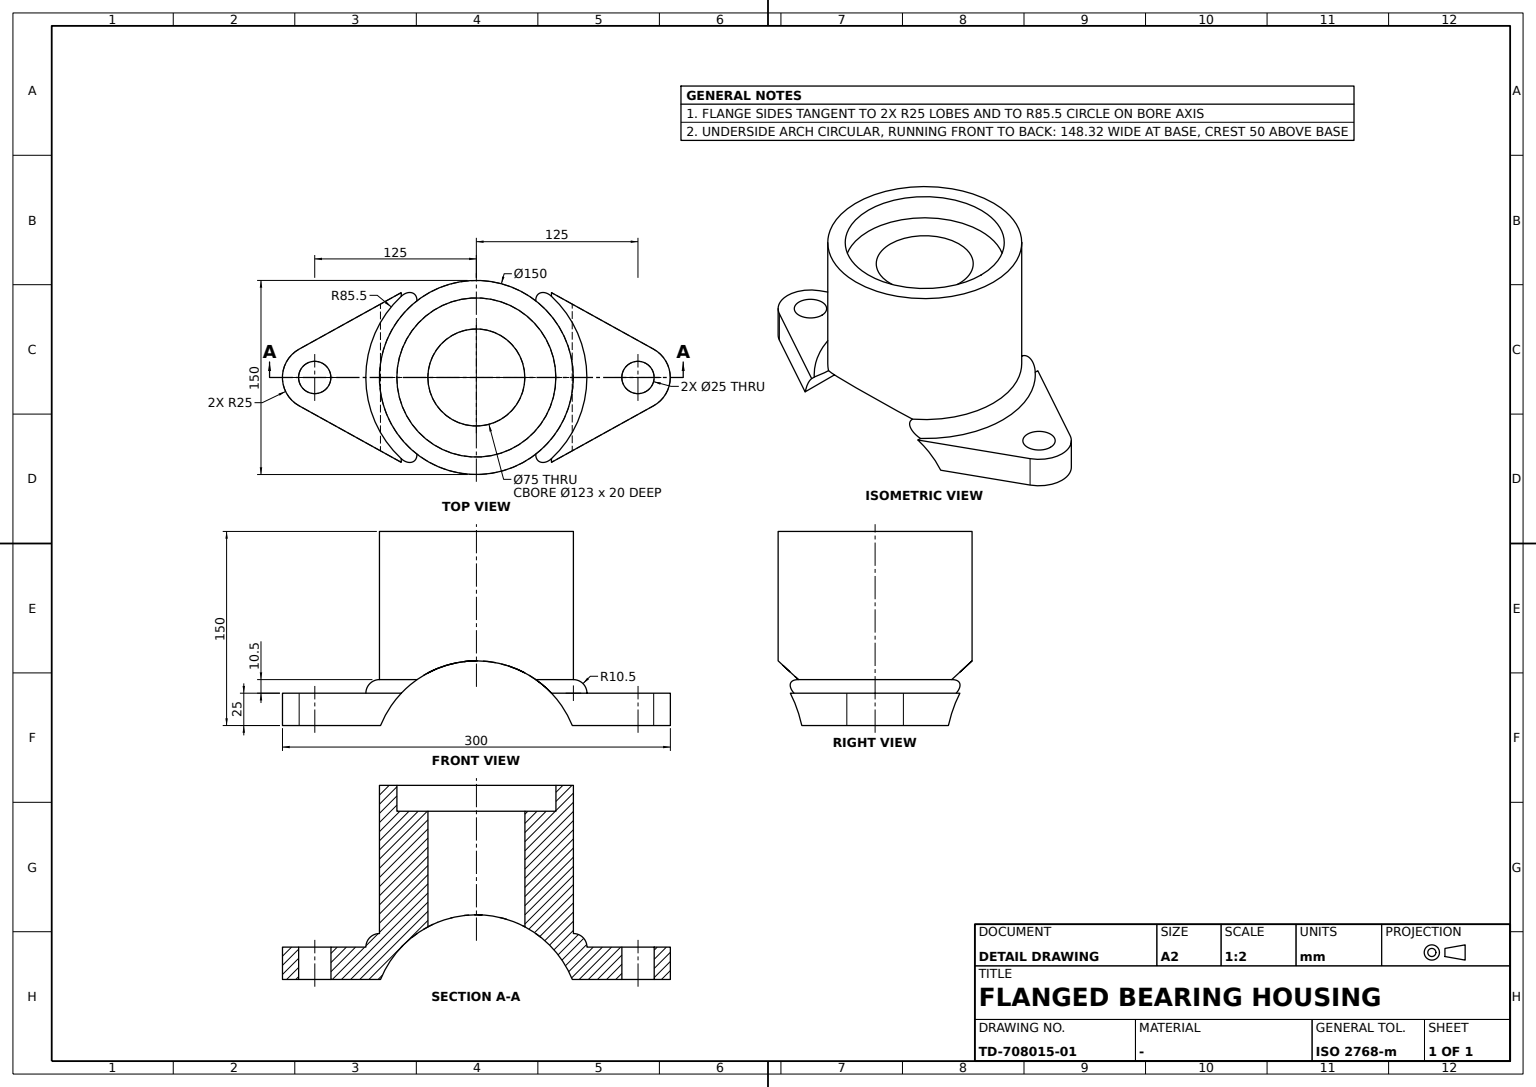
ISO-10303-21;
HEADER;
FILE_DESCRIPTION((''),'2;1');
FILE_NAME('','',(''),(''),'','','');
FILE_SCHEMA(('AUTOMOTIVE_DESIGN'));
ENDSEC;
DATA;
#1=APPLICATION_CONTEXT('');
#2=PRODUCT_CONTEXT('',#1,'mechanical');
#3=PRODUCT('','','',(#2));
#4=PRODUCT_DEFINITION_FORMATION('','',#3);
#5=PRODUCT_DEFINITION_CONTEXT('',#1,'design');
#6=PRODUCT_DEFINITION('','',#4,#5);
#7=PRODUCT_DEFINITION_SHAPE('','',#6);
#8=(LENGTH_UNIT()NAMED_UNIT(*)SI_UNIT(.MILLI.,.METRE.));
#9=(NAMED_UNIT(*)PLANE_ANGLE_UNIT()SI_UNIT($,.RADIAN.));
#10=(NAMED_UNIT(*)SI_UNIT($,.STERADIAN.)SOLID_ANGLE_UNIT());
#11=UNCERTAINTY_MEASURE_WITH_UNIT(LENGTH_MEASURE(1.E-05),#8,'distance_accuracy_value','');
#12=(GEOMETRIC_REPRESENTATION_CONTEXT(3)GLOBAL_UNCERTAINTY_ASSIGNED_CONTEXT((#11))GLOBAL_UNIT_ASSIGNED_CONTEXT((#8,#9,#10))REPRESENTATION_CONTEXT('',''));
#13=CARTESIAN_POINT('',(75.,0.,65.500023));
#14=VERTEX_POINT('',#13);
#15=CARTESIAN_POINT('',(45.932015,59.289544,65.500023));
#16=VERTEX_POINT('',#15);
#17=CARTESIAN_POINT('',(0.,0.,65.500023));
#18=DIRECTION('',(0.,0.,1.));
#19=DIRECTION('',(1.,0.,0.));
#20=AXIS2_PLACEMENT_3D('',#17,#18,#19);
#21=CIRCLE('',#20,75.);
#22=EDGE_CURVE('',#14,#16,#21,.T.);
#23=ORIENTED_EDGE('',*,*,#22,.T.);
#24=CARTESIAN_POINT('',(0.,74.999996,80.));
#25=VERTEX_POINT('',#24);
#26=CARTESIAN_POINT('',(44.42466,60.457302,66.557036));
#27=CARTESIAN_POINT('',(42.867243,61.587191,67.584494));
#28=CARTESIAN_POINT('',(41.259501,62.676771,68.579184));
#29=CARTESIAN_POINT('',(37.943975,64.769112,70.495736));
#30=CARTESIAN_POINT('',(34.432206,66.674154,72.251286));
#31=CARTESIAN_POINT('',(32.628216,67.576435,73.084976));
#32=CARTESIAN_POINT('',(28.788877,69.336495,74.71488));
#33=CARTESIAN_POINT('',(24.759204,70.848302,76.12074));
#34=CARTESIAN_POINT('',(22.623713,71.560134,76.783912));
#35=CARTESIAN_POINT('',(18.26572,72.83147,77.970027));
#36=CARTESIAN_POINT('',(13.757738,73.781552,78.858624));
#37=CARTESIAN_POINT('',(11.472246,74.17213,79.224278));
#38=CARTESIAN_POINT('',(7.811173,74.651918,79.673714));
#39=CARTESIAN_POINT('',(4.111316,74.906018,79.911892));
#40=CARTESIAN_POINT('',(2.741968,74.968674,79.970633));
#41=CARTESIAN_POINT('',(1.370943,74.999997,80.));
#42=B_SPLINE_CURVE_WITH_KNOTS('',5,(#15,#26,#27,#28,#29,#30,#31,#32,#33,#34,#35,#36,#37,#38,#39,#40,#41,#24),.UNSPECIFIED.,.F.,.F.,(6,3,3,3,3,6),(0.000015545,15.416004002,30.832008004,47.400792482,63.96957696,73.665798497),.UNSPECIFIED.);
#43=EDGE_CURVE('',#16,#25,#42,.T.);
#44=ORIENTED_EDGE('',*,*,#43,.T.);
#45=CARTESIAN_POINT('',(-35.956915,65.818692,71.463979));
#46=VERTEX_POINT('',#45);
#47=CARTESIAN_POINT('',(-3.005582,74.999994,80.));
#48=CARTESIAN_POINT('',(-6.010768,74.849434,79.858851));
#49=CARTESIAN_POINT('',(-8.997009,74.548401,79.576624));
#50=CARTESIAN_POINT('',(-13.856972,73.811882,78.886712));
#51=CARTESIAN_POINT('',(-18.575435,72.700605,77.84818));
#52=CARTESIAN_POINT('',(-20.404325,72.207987,77.388242));
#53=CARTESIAN_POINT('',(-24.004028,71.116214,76.370136));
#54=CARTESIAN_POINT('',(-27.477294,69.822077,75.166705));
#55=CARTESIAN_POINT('',(-29.179745,69.127095,74.521442));
#56=CARTESIAN_POINT('',(-31.57301,68.064182,73.536419));
#57=CARTESIAN_POINT('',(-33.889508,66.913561,72.473425));
#58=CARTESIAN_POINT('',(-34.586075,66.556124,72.143525));
#59=CARTESIAN_POINT('',(-35.275165,66.191134,71.807));
#60=B_SPLINE_CURVE_WITH_KNOTS('',5,(#24,#47,#48,#49,#50,#51,#52,#53,#54,#55,#56,#57,#58,#59,#45),.UNSPECIFIED.,.F.,.F.,(6,3,3,3,6),(73.665798497,94.92327613,108.689934936,122.456593742,128.461425552),.UNSPECIFIED.);
#61=EDGE_CURVE('',#25,#46,#60,.T.);
#62=ORIENTED_EDGE('',*,*,#61,.T.);
#63=CARTESIAN_POINT('',(-35.956915,65.818692,180.));
#64=VERTEX_POINT('',#63);
#65=CARTESIAN_POINT('',(-35.956915,65.818692,122.75));
#66=VECTOR('',#18,1000.);
#67=LINE('',#65,#66);
#68=EDGE_CURVE('',#46,#64,#67,.T.);
#69=ORIENTED_EDGE('',*,*,#68,.T.);
#70=CARTESIAN_POINT('',(75.,0.,180.));
#71=VERTEX_POINT('',#70);
#72=CARTESIAN_POINT('',(0.,0.,180.));
#73=AXIS2_PLACEMENT_3D('',#72,#18,#19);
#74=CIRCLE('',#73,75.);
#75=EDGE_CURVE('',#71,#64,#74,.T.);
#76=ORIENTED_EDGE('',*,*,#75,.F.);
#77=CARTESIAN_POINT('',(75.,0.,105.));
#78=DIRECTION('',(0.,0.,-1.));
#79=VECTOR('',#78,1000.);
#80=LINE('',#77,#79);
#81=EDGE_CURVE('',#71,#14,#80,.T.);
#82=ORIENTED_EDGE('',*,*,#81,.T.);
#83=EDGE_LOOP('',(#23,#44,#62,#69,#76,#82));
#84=FACE_OUTER_BOUND('',#83,.T.);
#85=CARTESIAN_POINT('',(0.,0.,105.));
#86=AXIS2_PLACEMENT_3D('',#85,#78,#19);
#87=CYLINDRICAL_SURFACE('',#86,75.);
#88=ADVANCED_FACE('',(#84),#87,.T.);
#89=CARTESIAN_POINT('',(137.5,0.,30.));
#90=VERTEX_POINT('',#89);
#91=CARTESIAN_POINT('',(137.5,0.,55.));
#92=VERTEX_POINT('',#91);
#93=CARTESIAN_POINT('',(137.5,0.,42.5));
#94=LINE('',#93,#66);
#95=EDGE_CURVE('',#90,#92,#94,.T.);
#96=ORIENTED_EDGE('',*,*,#95,.T.);
#97=CARTESIAN_POINT('',(112.5,0.,55.));
#98=VERTEX_POINT('',#97);
#99=CARTESIAN_POINT('',(125.,0.,55.));
#100=AXIS2_PLACEMENT_3D('',#99,#18,#19);
#101=CIRCLE('',#100,12.5);
#102=EDGE_CURVE('',#92,#98,#101,.T.);
#103=ORIENTED_EDGE('',*,*,#102,.T.);
#104=CARTESIAN_POINT('',(112.5,0.,30.));
#105=VERTEX_POINT('',#104);
#106=CARTESIAN_POINT('',(112.5,0.,42.5));
#107=LINE('',#106,#66);
#108=EDGE_CURVE('',#105,#98,#107,.T.);
#109=ORIENTED_EDGE('',*,*,#108,.F.);
#110=CARTESIAN_POINT('',(125.,0.,30.));
#111=AXIS2_PLACEMENT_3D('',#110,#18,#19);
#112=CIRCLE('',#111,12.5);
#113=EDGE_CURVE('',#90,#105,#112,.T.);
#114=ORIENTED_EDGE('',*,*,#113,.F.);
#115=EDGE_LOOP('',(#96,#103,#109,#114));
#116=FACE_OUTER_BOUND('',#115,.T.);
#117=CARTESIAN_POINT('',(125.,0.,42.5));
#118=AXIS2_PLACEMENT_3D('',#117,#78,#19);
#119=CYLINDRICAL_SURFACE('',#118,12.5);
#120=ADVANCED_FACE('',(#116),#119,.F.);
#121=CARTESIAN_POINT('',(85.5,0.,55.));
#122=VERTEX_POINT('',#121);
#123=CARTESIAN_POINT('',(58.09475,62.731571,55.));
#124=VERTEX_POINT('',#123);
#125=CARTESIAN_POINT('',(0.,0.,55.));
#126=AXIS2_PLACEMENT_3D('',#125,#18,#19);
#127=CIRCLE('',#126,85.5);
#128=EDGE_CURVE('',#122,#124,#127,.T.);
#129=ORIENTED_EDGE('',*,*,#128,.T.);
#130=CARTESIAN_POINT('',(45.931984,59.781253,65.500022));
#131=CARTESIAN_POINT('',(45.957633,60.273534,65.482035));
#132=CARTESIAN_POINT('',(46.013598,60.764433,65.442792));
#133=CARTESIAN_POINT('',(46.18265,61.650021,65.323969));
#134=CARTESIAN_POINT('',(46.482222,62.479557,65.111051));
#135=CARTESIAN_POINT('',(46.64702,62.840187,64.993318));
#136=CARTESIAN_POINT('',(47.027114,63.507624,64.719601));
#137=CARTESIAN_POINT('',(47.501145,64.072254,64.372156));
#138=CARTESIAN_POINT('',(47.754707,64.322458,64.184509));
#139=CARTESIAN_POINT('',(48.321137,64.788989,63.760572));
#140=CARTESIAN_POINT('',(48.939003,65.131341,63.286907));
#141=CARTESIAN_POINT('',(49.273241,65.278339,63.02718));
#142=CARTESIAN_POINT('',(50.019614,65.534776,62.438942));
#143=CARTESIAN_POINT('',(50.781809,65.657134,61.819435));
#144=CARTESIAN_POINT('',(51.197806,65.68824,61.475396));
#145=CARTESIAN_POINT('',(52.113214,65.686332,60.705115));
#146=CARTESIAN_POINT('',(53.012524,65.54194,59.919224));
#147=CARTESIAN_POINT('',(53.497419,65.425123,59.486573));
#148=CARTESIAN_POINT('',(54.531365,65.096952,58.545108));
#149=CARTESIAN_POINT('',(55.518174,64.620504,57.606723));
#150=CARTESIAN_POINT('',(56.035452,64.324691,57.103317));
#151=CARTESIAN_POINT('',(56.765953,63.84192,56.37648));
#152=CARTESIAN_POINT('',(57.461156,63.289923,55.662925));
#153=CARTESIAN_POINT('',(57.676041,63.109937,55.440197));
#154=CARTESIAN_POINT('',(57.887187,62.923792,55.219242));
#155=B_SPLINE_CURVE_WITH_KNOTS('',5,(#15,#130,#131,#132,#133,#134,#135,#136,#137,#138,#139,#140,#141,#142,#143,#144,#145,#146,#147,#148,#149,#150,#151,#152,#153,#154,#123),.UNSPECIFIED.,.F.,.F.,(6,3,3,3,3,3,3,3,6),(0.,3.476731119,6.383349563,9.21394229,12.349415898,16.103433711,20.647338583,25.97571507,28.413683168),.UNSPECIFIED.);
#156=EDGE_CURVE('',#16,#124,#155,.T.);
#157=ORIENTED_EDGE('',*,*,#156,.F.);
#158=ORIENTED_EDGE('',*,*,#22,.F.);
#159=CARTESIAN_POINT('',(74.999977,0.,55.));
#160=DIRECTION('',(0.,-1.,0.));
#161=AXIS2_PLACEMENT_3D('',#159,#160,#78);
#162=CIRCLE('',#161,10.500023);
#163=EDGE_CURVE('',#122,#14,#162,.T.);
#164=ORIENTED_EDGE('',*,*,#163,.F.);
#165=EDGE_LOOP('',(#129,#157,#158,#164));
#166=FACE_OUTER_BOUND('',#165,.T.);
#167=TOROIDAL_SURFACE('',#126,74.999977,10.500023);
#168=ADVANCED_FACE('',(#166),#167,.T.);
#169=CARTESIAN_POINT('',(-137.1,21.8767,30.));
#170=VERTEX_POINT('',#169);
#171=CARTESIAN_POINT('',(-137.1,21.8767,55.));
#172=VERTEX_POINT('',#171);
#173=CARTESIAN_POINT('',(-137.1,21.8767,42.5));
#174=LINE('',#173,#66);
#175=EDGE_CURVE('',#170,#172,#174,.T.);
#176=ORIENTED_EDGE('',*,*,#175,.F.);
#177=CARTESIAN_POINT('',(-137.1,-21.8767,30.));
#178=VERTEX_POINT('',#177);
#179=CARTESIAN_POINT('',(-125.,0.,30.));
#180=AXIS2_PLACEMENT_3D('',#179,#18,#19);
#181=CIRCLE('',#180,25.);
#182=EDGE_CURVE('',#170,#178,#181,.T.);
#183=ORIENTED_EDGE('',*,*,#182,.T.);
#184=CARTESIAN_POINT('',(-137.1,-21.8767,55.));
#185=VERTEX_POINT('',#184);
#186=CARTESIAN_POINT('',(-137.1,-21.8767,42.5));
#187=LINE('',#186,#66);
#188=EDGE_CURVE('',#178,#185,#187,.T.);
#189=ORIENTED_EDGE('',*,*,#188,.T.);
#190=CARTESIAN_POINT('',(-125.,0.,55.));
#191=AXIS2_PLACEMENT_3D('',#190,#18,#19);
#192=CIRCLE('',#191,25.);
#193=EDGE_CURVE('',#172,#185,#192,.T.);
#194=ORIENTED_EDGE('',*,*,#193,.F.);
#195=EDGE_LOOP('',(#176,#183,#189,#194));
#196=FACE_OUTER_BOUND('',#195,.T.);
#197=CARTESIAN_POINT('',(-125.,0.,42.5));
#198=AXIS2_PLACEMENT_3D('',#197,#78,#19);
#199=CYLINDRICAL_SURFACE('',#198,25.);
#200=ADVANCED_FACE('',(#196),#199,.T.);
#201=CARTESIAN_POINT('',(-58.09475,62.731571,55.));
#202=VERTEX_POINT('',#201);
#203=CARTESIAN_POINT('',(-58.09475,65.574494,55.));
#204=VERTEX_POINT('',#203);
#205=CARTESIAN_POINT('',(-58.09475,64.153032,55.));
#206=DIRECTION('',(0.,1.,0.));
#207=VECTOR('',#206,1000.);
#208=LINE('',#205,#207);
#209=EDGE_CURVE('',#202,#204,#208,.T.);
#210=ORIENTED_EDGE('',*,*,#209,.T.);
#211=CARTESIAN_POINT('',(-97.597375,43.725597,55.));
#212=DIRECTION('',(-0.875067997,-0.484,0.));
#213=VECTOR('',#212,1000.);
#214=LINE('',#211,#213);
#215=EDGE_CURVE('',#204,#172,#214,.T.);
#216=ORIENTED_EDGE('',*,*,#215,.T.);
#217=ORIENTED_EDGE('',*,*,#193,.T.);
#218=CARTESIAN_POINT('',(-58.09475,-65.574494,55.));
#219=VERTEX_POINT('',#218);
#220=CARTESIAN_POINT('',(-97.597375,-43.725597,55.));
#221=DIRECTION('',(0.875067997,-0.484,0.));
#222=VECTOR('',#221,1000.);
#223=LINE('',#220,#222);
#224=EDGE_CURVE('',#185,#219,#223,.T.);
#225=ORIENTED_EDGE('',*,*,#224,.T.);
#226=CARTESIAN_POINT('',(-58.09475,-62.731571,55.));
#227=VERTEX_POINT('',#226);
#228=CARTESIAN_POINT('',(-58.09475,-64.153032,55.));
#229=LINE('',#228,#207);
#230=EDGE_CURVE('',#219,#227,#229,.T.);
#231=ORIENTED_EDGE('',*,*,#230,.T.);
#232=EDGE_CURVE('',#202,#227,#127,.T.);
#233=ORIENTED_EDGE('',*,*,#232,.F.);
#234=EDGE_LOOP('',(#210,#216,#217,#225,#231,#233));
#235=FACE_OUTER_BOUND('',#234,.T.);
#236=CARTESIAN_POINT('',(-137.5,0.,55.));
#237=VERTEX_POINT('',#236);
#238=CARTESIAN_POINT('',(-112.5,0.,55.));
#239=VERTEX_POINT('',#238);
#240=CIRCLE('',#191,12.5);
#241=EDGE_CURVE('',#237,#239,#240,.T.);
#242=ORIENTED_EDGE('',*,*,#241,.F.);
#243=EDGE_CURVE('',#239,#237,#240,.T.);
#244=ORIENTED_EDGE('',*,*,#243,.F.);
#245=EDGE_LOOP('',(#242,#244));
#246=FACE_BOUND('',#245,.T.);
#247=PLANE('',#126);
#248=ADVANCED_FACE('',(#235,#246),#247,.T.);
#249=ORIENTED_EDGE('',*,*,#113,.T.);
#250=EDGE_CURVE('',#105,#90,#112,.T.);
#251=ORIENTED_EDGE('',*,*,#250,.T.);
#252=EDGE_LOOP('',(#249,#251));
#253=FACE_BOUND('',#252,.T.);
#254=CARTESIAN_POINT('',(137.1,-21.8767,30.));
#255=VERTEX_POINT('',#254);
#256=CARTESIAN_POINT('',(150.,0.,30.));
#257=VERTEX_POINT('',#256);
#258=CIRCLE('',#111,25.);
#259=EDGE_CURVE('',#255,#257,#258,.T.);
#260=ORIENTED_EDGE('',*,*,#259,.F.);
#261=CARTESIAN_POINT('',(74.161985,-56.687708,30.));
#262=VERTEX_POINT('',#261);
#263=CARTESIAN_POINT('',(105.630992,-39.282204,30.));
#264=DIRECTION('',(0.875067997,0.484,0.));
#265=VECTOR('',#264,1000.);
#266=LINE('',#263,#265);
#267=EDGE_CURVE('',#262,#255,#266,.T.);
#268=ORIENTED_EDGE('',*,*,#267,.F.);
#269=CARTESIAN_POINT('',(74.161985,56.687708,30.));
#270=VERTEX_POINT('',#269);
#271=CARTESIAN_POINT('',(74.161985,0.,30.));
#272=LINE('',#271,#207);
#273=EDGE_CURVE('',#262,#270,#272,.T.);
#274=ORIENTED_EDGE('',*,*,#273,.T.);
#275=CARTESIAN_POINT('',(137.1,21.8767,30.));
#276=VERTEX_POINT('',#275);
#277=CARTESIAN_POINT('',(105.630992,39.282204,30.));
#278=DIRECTION('',(-0.875067997,0.484,0.));
#279=VECTOR('',#278,1000.);
#280=LINE('',#277,#279);
#281=EDGE_CURVE('',#276,#270,#280,.T.);
#282=ORIENTED_EDGE('',*,*,#281,.F.);
#283=EDGE_CURVE('',#257,#276,#258,.T.);
#284=ORIENTED_EDGE('',*,*,#283,.F.);
#285=EDGE_LOOP('',(#260,#268,#274,#282,#284));
#286=FACE_OUTER_BOUND('',#285,.T.);
#287=CARTESIAN_POINT('',(0.,0.,30.));
#288=AXIS2_PLACEMENT_3D('',#287,#18,#19);
#289=PLANE('',#288);
#290=ADVANCED_FACE('',(#253,#286),#289,.F.);
#291=ORIENTED_EDGE('',*,*,#267,.T.);
#292=CARTESIAN_POINT('',(137.1,-21.8767,55.));
#293=VERTEX_POINT('',#292);
#294=CARTESIAN_POINT('',(137.1,-21.8767,42.5));
#295=LINE('',#294,#66);
#296=EDGE_CURVE('',#255,#293,#295,.T.);
#297=ORIENTED_EDGE('',*,*,#296,.T.);
#298=CARTESIAN_POINT('',(58.09475,-65.574494,55.));
#299=VERTEX_POINT('',#298);
#300=CARTESIAN_POINT('',(97.597375,-43.725597,55.));
#301=LINE('',#300,#265);
#302=EDGE_CURVE('',#299,#293,#301,.T.);
#303=ORIENTED_EDGE('',*,*,#302,.F.);
#304=CARTESIAN_POINT('',(72.651421,-57.523201,33.734213));
#305=CARTESIAN_POINT('',(70.91552,-58.483328,37.349387));
#306=CARTESIAN_POINT('',(68.969618,-59.559605,40.824944));
#307=CARTESIAN_POINT('',(65.725248,-61.354066,45.863813));
#308=CARTESIAN_POINT('',(62.07998,-63.370264,50.518882));
#309=CARTESIAN_POINT('',(60.792453,-64.082395,52.060452));
#310=CARTESIAN_POINT('',(59.463241,-64.817582,53.554507));
#311=B_SPLINE_CURVE_WITH_KNOTS('',5,(#261,#304,#305,#306,#307,#308,#309,#310,#298),.UNSPECIFIED.,.F.,.F.,(6,3,6),(0.,29.089689473,44.1481303),.UNSPECIFIED.);
#312=EDGE_CURVE('',#262,#299,#311,.T.);
#313=ORIENTED_EDGE('',*,*,#312,.F.);
#314=EDGE_LOOP('',(#291,#297,#303,#313));
#315=FACE_OUTER_BOUND('',#314,.T.);
#316=DIRECTION('',(-0.484,0.875067997,0.));
#317=AXIS2_PLACEMENT_3D('',#254,#316,#212);
#318=PLANE('',#317);
#319=ADVANCED_FACE('',(#315),#318,.F.);
#320=CARTESIAN_POINT('',(-61.5,0.,160.));
#321=VERTEX_POINT('',#320);
#322=CARTESIAN_POINT('',(61.5,0.,160.));
#323=VERTEX_POINT('',#322);
#324=CARTESIAN_POINT('',(0.,0.,160.));
#325=AXIS2_PLACEMENT_3D('',#324,#18,#19);
#326=CIRCLE('',#325,61.5);
#327=EDGE_CURVE('',#321,#323,#326,.T.);
#328=ORIENTED_EDGE('',*,*,#327,.T.);
#329=EDGE_CURVE('',#323,#321,#326,.T.);
#330=ORIENTED_EDGE('',*,*,#329,.T.);
#331=EDGE_LOOP('',(#328,#330));
#332=FACE_OUTER_BOUND('',#331,.T.);
#333=CARTESIAN_POINT('',(-37.5,0.,160.));
#334=VERTEX_POINT('',#333);
#335=CARTESIAN_POINT('',(37.5,0.,160.));
#336=VERTEX_POINT('',#335);
#337=AXIS2_PLACEMENT_3D('',#324,#78,#19);
#338=CIRCLE('',#337,37.5);
#339=EDGE_CURVE('',#334,#336,#338,.T.);
#340=ORIENTED_EDGE('',*,*,#339,.T.);
#341=EDGE_CURVE('',#336,#334,#338,.T.);
#342=ORIENTED_EDGE('',*,*,#341,.T.);
#343=EDGE_LOOP('',(#340,#342));
#344=FACE_BOUND('',#343,.T.);
#345=PLANE('',#325);
#346=ADVANCED_FACE('',(#332,#344),#345,.T.);
#347=ORIENTED_EDGE('',*,*,#188,.F.);
#348=CARTESIAN_POINT('',(-74.161985,-56.687708,30.));
#349=VERTEX_POINT('',#348);
#350=CARTESIAN_POINT('',(-105.630992,-39.282204,30.));
#351=LINE('',#350,#222);
#352=EDGE_CURVE('',#178,#349,#351,.T.);
#353=ORIENTED_EDGE('',*,*,#352,.T.);
#354=CARTESIAN_POINT('',(-72.651421,-57.523201,33.734213));
#355=CARTESIAN_POINT('',(-70.91552,-58.483328,37.349387));
#356=CARTESIAN_POINT('',(-68.969618,-59.559605,40.824944));
#357=CARTESIAN_POINT('',(-65.725248,-61.354066,45.863813));
#358=CARTESIAN_POINT('',(-62.07998,-63.370264,50.518882));
#359=CARTESIAN_POINT('',(-60.792453,-64.082395,52.060452));
#360=CARTESIAN_POINT('',(-59.463241,-64.817582,53.554507));
#361=B_SPLINE_CURVE_WITH_KNOTS('',5,(#348,#354,#355,#356,#357,#358,#359,#360,#218),.UNSPECIFIED.,.F.,.F.,(6,3,6),(0.,29.08968947,44.148130297),.UNSPECIFIED.);
#362=EDGE_CURVE('',#349,#219,#361,.T.);
#363=ORIENTED_EDGE('',*,*,#362,.T.);
#364=ORIENTED_EDGE('',*,*,#224,.F.);
#365=EDGE_LOOP('',(#347,#353,#363,#364));
#366=FACE_OUTER_BOUND('',#365,.T.);
#367=DIRECTION('',(-0.484,-0.875067997,0.));
#368=AXIS2_PLACEMENT_3D('',#177,#367,#221);
#369=PLANE('',#368);
#370=ADVANCED_FACE('',(#366),#369,.T.);
#371=CARTESIAN_POINT('',(61.5,0.,180.));
#372=VERTEX_POINT('',#371);
#373=CARTESIAN_POINT('',(-61.5,0.,180.));
#374=VERTEX_POINT('',#373);
#375=CIRCLE('',#73,61.5);
#376=EDGE_CURVE('',#372,#374,#375,.T.);
#377=ORIENTED_EDGE('',*,*,#376,.F.);
#378=EDGE_CURVE('',#374,#372,#375,.T.);
#379=ORIENTED_EDGE('',*,*,#378,.F.);
#380=EDGE_LOOP('',(#377,#379));
#381=FACE_BOUND('',#380,.T.);
#382=ORIENTED_EDGE('',*,*,#75,.T.);
#383=CARTESIAN_POINT('',(35.956915,-65.818692,180.));
#384=VERTEX_POINT('',#383);
#385=EDGE_CURVE('',#64,#384,#74,.T.);
#386=ORIENTED_EDGE('',*,*,#385,.T.);
#387=EDGE_CURVE('',#384,#71,#74,.T.);
#388=ORIENTED_EDGE('',*,*,#387,.T.);
#389=EDGE_LOOP('',(#382,#386,#388));
#390=FACE_OUTER_BOUND('',#389,.T.);
#391=PLANE('',#73);
#392=ADVANCED_FACE('',(#381,#390),#391,.T.);
#393=CARTESIAN_POINT('',(58.09475,65.574494,55.));
#394=VERTEX_POINT('',#393);
#395=CARTESIAN_POINT('',(72.651421,57.523201,33.734213));
#396=CARTESIAN_POINT('',(70.91552,58.483328,37.349387));
#397=CARTESIAN_POINT('',(68.969618,59.559605,40.824944));
#398=CARTESIAN_POINT('',(65.725248,61.354066,45.863813));
#399=CARTESIAN_POINT('',(62.07998,63.370264,50.518882));
#400=CARTESIAN_POINT('',(60.792453,64.082395,52.060452));
#401=CARTESIAN_POINT('',(59.463241,64.817582,53.554507));
#402=B_SPLINE_CURVE_WITH_KNOTS('',5,(#269,#395,#396,#397,#398,#399,#400,#401,#393),.UNSPECIFIED.,.F.,.F.,(6,3,6),(0.,29.089689473,44.1481303),.UNSPECIFIED.);
#403=EDGE_CURVE('',#270,#394,#402,.T.);
#404=ORIENTED_EDGE('',*,*,#403,.T.);
#405=CARTESIAN_POINT('',(137.1,21.8767,55.));
#406=VERTEX_POINT('',#405);
#407=CARTESIAN_POINT('',(97.597375,43.725597,55.));
#408=LINE('',#407,#279);
#409=EDGE_CURVE('',#406,#394,#408,.T.);
#410=ORIENTED_EDGE('',*,*,#409,.F.);
#411=CARTESIAN_POINT('',(137.1,21.8767,42.5));
#412=LINE('',#411,#66);
#413=EDGE_CURVE('',#276,#406,#412,.T.);
#414=ORIENTED_EDGE('',*,*,#413,.F.);
#415=ORIENTED_EDGE('',*,*,#281,.T.);
#416=EDGE_LOOP('',(#404,#410,#414,#415));
#417=FACE_OUTER_BOUND('',#416,.T.);
#418=DIRECTION('',(0.484,0.875067997,0.));
#419=AXIS2_PLACEMENT_3D('',#275,#418,#278);
#420=PLANE('',#419);
#421=ADVANCED_FACE('',(#417),#420,.T.);
#422=CARTESIAN_POINT('',(45.932015,-59.289544,65.500023));
#423=VERTEX_POINT('',#422);
#424=EDGE_CURVE('',#423,#14,#21,.T.);
#425=ORIENTED_EDGE('',*,*,#424,.F.);
#426=CARTESIAN_POINT('',(58.09475,-62.731571,55.));
#427=VERTEX_POINT('',#426);
#428=CARTESIAN_POINT('',(45.931984,-59.781253,65.500022));
#429=CARTESIAN_POINT('',(45.957633,-60.273534,65.482035));
#430=CARTESIAN_POINT('',(46.013598,-60.764433,65.442792));
#431=CARTESIAN_POINT('',(46.18265,-61.650021,65.323969));
#432=CARTESIAN_POINT('',(46.482222,-62.479557,65.111051));
#433=CARTESIAN_POINT('',(46.64702,-62.840187,64.993318));
#434=CARTESIAN_POINT('',(47.027114,-63.507624,64.719601));
#435=CARTESIAN_POINT('',(47.501145,-64.072254,64.372156));
#436=CARTESIAN_POINT('',(47.754707,-64.322458,64.184509));
#437=CARTESIAN_POINT('',(48.321137,-64.788989,63.760572));
#438=CARTESIAN_POINT('',(48.939003,-65.131341,63.286907));
#439=CARTESIAN_POINT('',(49.273241,-65.278339,63.02718));
#440=CARTESIAN_POINT('',(50.019614,-65.534776,62.438942));
#441=CARTESIAN_POINT('',(50.781809,-65.657134,61.819435));
#442=CARTESIAN_POINT('',(51.197806,-65.68824,61.475396));
#443=CARTESIAN_POINT('',(52.113214,-65.686332,60.705115));
#444=CARTESIAN_POINT('',(53.012524,-65.54194,59.919224));
#445=CARTESIAN_POINT('',(53.497419,-65.425123,59.486573));
#446=CARTESIAN_POINT('',(54.531365,-65.096952,58.545108));
#447=CARTESIAN_POINT('',(55.518174,-64.620504,57.606723));
#448=CARTESIAN_POINT('',(56.035452,-64.324691,57.103317));
#449=CARTESIAN_POINT('',(56.765953,-63.84192,56.37648));
#450=CARTESIAN_POINT('',(57.461156,-63.289923,55.662925));
#451=CARTESIAN_POINT('',(57.676041,-63.109937,55.440197));
#452=CARTESIAN_POINT('',(57.887187,-62.923792,55.219242));
#453=B_SPLINE_CURVE_WITH_KNOTS('',5,(#422,#428,#429,#430,#431,#432,#433,#434,#435,#436,#437,#438,#439,#440,#441,#442,#443,#444,#445,#446,#447,#448,#449,#450,#451,#452,#426),.UNSPECIFIED.,.F.,.F.,(6,3,3,3,3,3,3,3,6),(0.,3.476731118,6.383349561,9.213942288,12.349415895,16.103433708,20.647338579,25.975715066,28.413683166),.UNSPECIFIED.);
#454=EDGE_CURVE('',#423,#427,#453,.T.);
#455=ORIENTED_EDGE('',*,*,#454,.T.);
#456=EDGE_CURVE('',#427,#122,#127,.T.);
#457=ORIENTED_EDGE('',*,*,#456,.T.);
#458=ORIENTED_EDGE('',*,*,#163,.T.);
#459=EDGE_LOOP('',(#425,#455,#457,#458));
#460=FACE_OUTER_BOUND('',#459,.T.);
#461=ADVANCED_FACE('',(#460),#167,.T.);
#462=ORIENTED_EDGE('',*,*,#108,.T.);
#463=EDGE_CURVE('',#98,#92,#101,.T.);
#464=ORIENTED_EDGE('',*,*,#463,.T.);
#465=ORIENTED_EDGE('',*,*,#95,.F.);
#466=ORIENTED_EDGE('',*,*,#250,.F.);
#467=EDGE_LOOP('',(#462,#464,#465,#466));
#468=FACE_OUTER_BOUND('',#467,.T.);
#469=ADVANCED_FACE('',(#468),#119,.F.);
#470=ORIENTED_EDGE('',*,*,#413,.T.);
#471=CARTESIAN_POINT('',(150.,0.,55.));
#472=VERTEX_POINT('',#471);
#473=CIRCLE('',#100,25.);
#474=EDGE_CURVE('',#472,#406,#473,.T.);
#475=ORIENTED_EDGE('',*,*,#474,.F.);
#476=CARTESIAN_POINT('',(150.,0.,42.5));
#477=LINE('',#476,#79);
#478=EDGE_CURVE('',#472,#257,#477,.T.);
#479=ORIENTED_EDGE('',*,*,#478,.T.);
#480=ORIENTED_EDGE('',*,*,#283,.T.);
#481=EDGE_LOOP('',(#470,#475,#479,#480));
#482=FACE_OUTER_BOUND('',#481,.T.);
#483=CYLINDRICAL_SURFACE('',#118,25.);
#484=ADVANCED_FACE('',(#482),#483,.T.);
#485=ORIENTED_EDGE('',*,*,#243,.T.);
#486=CARTESIAN_POINT('',(-137.5,0.,30.));
#487=VERTEX_POINT('',#486);
#488=CARTESIAN_POINT('',(-137.5,0.,42.5));
#489=LINE('',#488,#66);
#490=EDGE_CURVE('',#487,#237,#489,.T.);
#491=ORIENTED_EDGE('',*,*,#490,.F.);
#492=CARTESIAN_POINT('',(-112.5,0.,30.));
#493=VERTEX_POINT('',#492);
#494=CIRCLE('',#180,12.5);
#495=EDGE_CURVE('',#493,#487,#494,.T.);
#496=ORIENTED_EDGE('',*,*,#495,.F.);
#497=CARTESIAN_POINT('',(-112.5,0.,42.5));
#498=LINE('',#497,#66);
#499=EDGE_CURVE('',#493,#239,#498,.T.);
#500=ORIENTED_EDGE('',*,*,#499,.T.);
#501=EDGE_LOOP('',(#485,#491,#496,#500));
#502=FACE_OUTER_BOUND('',#501,.T.);
#503=CYLINDRICAL_SURFACE('',#198,12.5);
#504=ADVANCED_FACE('',(#502),#503,.F.);
#505=CARTESIAN_POINT('',(0.,-74.999996,80.));
#506=VERTEX_POINT('',#505);
#507=CARTESIAN_POINT('',(35.956915,-65.818692,71.463979));
#508=VERTEX_POINT('',#507);
#509=CARTESIAN_POINT('',(3.005582,-74.999994,80.));
#510=CARTESIAN_POINT('',(6.010768,-74.849434,79.858851));
#511=CARTESIAN_POINT('',(8.997009,-74.548401,79.576624));
#512=CARTESIAN_POINT('',(13.856972,-73.811882,78.886712));
#513=CARTESIAN_POINT('',(18.575435,-72.700605,77.84818));
#514=CARTESIAN_POINT('',(20.404325,-72.207987,77.388242));
#515=CARTESIAN_POINT('',(24.004028,-71.116214,76.370136));
#516=CARTESIAN_POINT('',(27.477294,-69.822077,75.166705));
#517=CARTESIAN_POINT('',(29.179745,-69.127095,74.521442));
#518=CARTESIAN_POINT('',(31.573042,-68.064168,73.536405));
#519=CARTESIAN_POINT('',(33.889571,-66.913529,72.473396));
#520=CARTESIAN_POINT('',(34.58597,-66.556179,72.143577));
#521=CARTESIAN_POINT('',(35.275108,-66.191165,71.807028));
#522=B_SPLINE_CURVE_WITH_KNOTS('',5,(#505,#509,#510,#511,#512,#513,#514,#515,#516,#517,#518,#519,#520,#521,#507),.UNSPECIFIED.,.F.,.F.,(6,3,3,3,6),(73.665798504,94.923276133,108.689934939,122.456593745,128.461693323),.UNSPECIFIED.);
#523=EDGE_CURVE('',#506,#508,#522,.T.);
#524=ORIENTED_EDGE('',*,*,#523,.T.);
#525=CARTESIAN_POINT('',(35.956915,-65.818692,122.75));
#526=LINE('',#525,#66);
#527=EDGE_CURVE('',#508,#384,#526,.T.);
#528=ORIENTED_EDGE('',*,*,#527,.T.);
#529=ORIENTED_EDGE('',*,*,#385,.F.);
#530=ORIENTED_EDGE('',*,*,#68,.F.);
#531=CARTESIAN_POINT('',(-45.932015,59.289544,65.500023));
#532=VERTEX_POINT('',#531);
#533=CARTESIAN_POINT('',(-43.625146,61.076691,67.117697));
#534=CARTESIAN_POINT('',(-41.193211,62.7693,68.66155));
#535=CARTESIAN_POINT('',(-38.635493,64.355379,70.116259));
#536=B_SPLINE_CURVE_WITH_KNOTS('',4,(#531,#533,#534,#535,#45),.UNSPECIFIED.,.F.,.F.,(5,5),(0.000015545,18.874260923),.UNSPECIFIED.);
#537=EDGE_CURVE('',#532,#46,#536,.T.);
#538=ORIENTED_EDGE('',*,*,#537,.F.);
#539=CARTESIAN_POINT('',(-45.932015,-59.289544,65.500023));
#540=VERTEX_POINT('',#539);
#541=EDGE_CURVE('',#532,#540,#21,.T.);
#542=ORIENTED_EDGE('',*,*,#541,.T.);
#543=CARTESIAN_POINT('',(-44.42466,-60.457302,66.557036));
#544=CARTESIAN_POINT('',(-42.867243,-61.587191,67.584494));
#545=CARTESIAN_POINT('',(-41.259501,-62.676771,68.579184));
#546=CARTESIAN_POINT('',(-37.943975,-64.769112,70.495736));
#547=CARTESIAN_POINT('',(-34.432206,-66.674154,72.251286));
#548=CARTESIAN_POINT('',(-32.628216,-67.576435,73.084976));
#549=CARTESIAN_POINT('',(-28.788877,-69.336495,74.71488));
#550=CARTESIAN_POINT('',(-24.759204,-70.848302,76.12074));
#551=CARTESIAN_POINT('',(-22.623713,-71.560134,76.783912));
#552=CARTESIAN_POINT('',(-18.26572,-72.83147,77.970027));
#553=CARTESIAN_POINT('',(-13.757738,-73.781552,78.858624));
#554=CARTESIAN_POINT('',(-11.472246,-74.17213,79.224278));
#555=CARTESIAN_POINT('',(-7.811173,-74.651918,79.673714));
#556=CARTESIAN_POINT('',(-4.111316,-74.906018,79.911892));
#557=CARTESIAN_POINT('',(-2.741968,-74.968674,79.970633));
#558=CARTESIAN_POINT('',(-1.370943,-74.999997,80.));
#559=B_SPLINE_CURVE_WITH_KNOTS('',5,(#539,#543,#544,#545,#546,#547,#548,#549,#550,#551,#552,#553,#554,#555,#556,#557,#558,#505),.UNSPECIFIED.,.F.,.F.,(6,3,3,3,3,6),(0.000015545,15.416004003,30.832008005,47.400792484,63.969576964,73.665798504),.UNSPECIFIED.);
#560=EDGE_CURVE('',#540,#506,#559,.T.);
#561=ORIENTED_EDGE('',*,*,#560,.T.);
#562=EDGE_LOOP('',(#524,#528,#529,#530,#538,#542,#561));
#563=FACE_OUTER_BOUND('',#562,.T.);
#564=ADVANCED_FACE('',(#563),#87,.T.);
#565=EDGE_CURVE('',#487,#493,#494,.T.);
#566=ORIENTED_EDGE('',*,*,#565,.T.);
#567=ORIENTED_EDGE('',*,*,#495,.T.);
#568=EDGE_LOOP('',(#566,#567));
#569=FACE_BOUND('',#568,.T.);
#570=ORIENTED_EDGE('',*,*,#182,.F.);
#571=CARTESIAN_POINT('',(-74.161985,56.687708,30.));
#572=VERTEX_POINT('',#571);
#573=CARTESIAN_POINT('',(-105.630992,39.282204,30.));
#574=LINE('',#573,#213);
#575=EDGE_CURVE('',#572,#170,#574,.T.);
#576=ORIENTED_EDGE('',*,*,#575,.F.);
#577=CARTESIAN_POINT('',(-74.161985,0.,30.));
#578=LINE('',#577,#207);
#579=EDGE_CURVE('',#349,#572,#578,.T.);
#580=ORIENTED_EDGE('',*,*,#579,.F.);
#581=ORIENTED_EDGE('',*,*,#352,.F.);
#582=EDGE_LOOP('',(#570,#576,#580,#581));
#583=FACE_OUTER_BOUND('',#582,.T.);
#584=ADVANCED_FACE('',(#569,#583),#289,.F.);
#585=ORIENTED_EDGE('',*,*,#81,.F.);
#586=ORIENTED_EDGE('',*,*,#387,.F.);
#587=ORIENTED_EDGE('',*,*,#527,.F.);
#588=CARTESIAN_POINT('',(38.635503,-64.355371,70.116254));
#589=CARTESIAN_POINT('',(41.193375,-62.769196,68.661456));
#590=CARTESIAN_POINT('',(43.625222,-61.076631,67.117643));
#591=B_SPLINE_CURVE_WITH_KNOTS('',4,(#507,#588,#589,#590,#422),.UNSPECIFIED.,.F.,.F.,(5,5),(128.461693323,147.335310383),.UNSPECIFIED.);
#592=EDGE_CURVE('',#508,#423,#591,.T.);
#593=ORIENTED_EDGE('',*,*,#592,.T.);
#594=ORIENTED_EDGE('',*,*,#424,.T.);
#595=EDGE_LOOP('',(#585,#586,#587,#593,#594));
#596=FACE_OUTER_BOUND('',#595,.T.);
#597=ADVANCED_FACE('',(#596),#87,.T.);
#598=ORIENTED_EDGE('',*,*,#302,.T.);
#599=EDGE_CURVE('',#293,#472,#473,.T.);
#600=ORIENTED_EDGE('',*,*,#599,.T.);
#601=ORIENTED_EDGE('',*,*,#474,.T.);
#602=ORIENTED_EDGE('',*,*,#409,.T.);
#603=CARTESIAN_POINT('',(58.09475,64.153032,55.));
#604=LINE('',#603,#207);
#605=EDGE_CURVE('',#124,#394,#604,.T.);
#606=ORIENTED_EDGE('',*,*,#605,.F.);
#607=ORIENTED_EDGE('',*,*,#128,.F.);
#608=ORIENTED_EDGE('',*,*,#456,.F.);
#609=CARTESIAN_POINT('',(58.09475,-64.153032,55.));
#610=LINE('',#609,#207);
#611=EDGE_CURVE('',#299,#427,#610,.T.);
#612=ORIENTED_EDGE('',*,*,#611,.F.);
#613=EDGE_LOOP('',(#598,#600,#601,#602,#606,#607,#608,#612));
#614=FACE_OUTER_BOUND('',#613,.T.);
#615=ORIENTED_EDGE('',*,*,#463,.F.);
#616=ORIENTED_EDGE('',*,*,#102,.F.);
#617=EDGE_LOOP('',(#615,#616));
#618=FACE_BOUND('',#617,.T.);
#619=ADVANCED_FACE('',(#614,#618),#247,.T.);
#620=ORIENTED_EDGE('',*,*,#341,.F.);
#621=CARTESIAN_POINT('',(37.5,0.,70.66647));
#622=VERTEX_POINT('',#621);
#623=CARTESIAN_POINT('',(37.5,0.,104.34));
#624=LINE('',#623,#79);
#625=EDGE_CURVE('',#336,#622,#624,.T.);
#626=ORIENTED_EDGE('',*,*,#625,.T.);
#627=CARTESIAN_POINT('',(0.,-37.5,80.));
#628=VERTEX_POINT('',#627);
#629=CARTESIAN_POINT('',(0.738234,-37.5,80.));
#630=CARTESIAN_POINT('',(1.476487,-37.481834,79.991485));
#631=CARTESIAN_POINT('',(2.214038,-37.445499,79.974453));
#632=CARTESIAN_POINT('',(5.26077,-37.220133,79.868946));
#633=CARTESIAN_POINT('',(8.27046,-36.686312,79.620498));
#634=CARTESIAN_POINT('',(10.50947,-36.10741,79.353397));
#635=CARTESIAN_POINT('',(14.976787,-34.579184,78.662156));
#636=CARTESIAN_POINT('',(19.116617,-32.394494,77.72703));
#637=CARTESIAN_POINT('',(21.13636,-31.112681,77.196972));
#638=CARTESIAN_POINT('',(24.830481,-28.336453,76.102982));
#639=CARTESIAN_POINT('',(28.046945,-25.041399,74.948644));
#640=CARTESIAN_POINT('',(29.485312,-23.331097,74.389484));
#641=CARTESIAN_POINT('',(31.922098,-19.953516,73.37912));
#642=CARTESIAN_POINT('',(33.87897,-16.251334,72.481622));
#643=CARTESIAN_POINT('',(34.676434,-14.474241,72.100535));
#644=CARTESIAN_POINT('',(36.115083,-10.612942,71.392179));
#645=CARTESIAN_POINT('',(37.019467,-6.555707,70.921535));
#646=CARTESIAN_POINT('',(37.339815,-4.38431,70.751474));
#647=CARTESIAN_POINT('',(37.5,-2.192155,70.66647));
#648=B_SPLINE_CURVE_WITH_KNOTS('',5,(#627,#629,#630,#631,#632,#633,#634,#635,#636,#637,#638,#639,#640,#641,#642,#643,#644,#645,#646,#647,#621),.UNSPECIFIED.,.F.,.F.,(6,3,3,3,3,3,6),(253.735689324,258.956265706,275.343173087,292.592813505,308.822862181,322.813937441,338.314815621),.UNSPECIFIED.);
#649=EDGE_CURVE('',#628,#622,#648,.T.);
#650=ORIENTED_EDGE('',*,*,#649,.F.);
#651=CARTESIAN_POINT('',(-37.5,0.,70.66647));
#652=VERTEX_POINT('',#651);
#653=CARTESIAN_POINT('',(-37.499999,-0.895469,70.66647));
#654=CARTESIAN_POINT('',(-37.473271,-1.790939,70.680654));
#655=CARTESIAN_POINT('',(-37.419814,-2.685068,70.709022));
#656=CARTESIAN_POINT('',(-37.142802,-5.769617,70.855569));
#657=CARTESIAN_POINT('',(-36.550455,-8.806099,71.164877));
#658=CARTESIAN_POINT('',(-35.973738,-10.921314,71.461317));
#659=CARTESIAN_POINT('',(-34.667508,-14.629294,72.11169));
#660=CARTESIAN_POINT('',(-32.907898,-18.105963,72.926392));
#661=CARTESIAN_POINT('',(-32.038026,-19.603156,73.314957));
#662=CARTESIAN_POINT('',(-29.521191,-23.413681,74.390333));
#663=CARTESIAN_POINT('',(-26.461469,-26.796646,75.54035));
#664=CARTESIAN_POINT('',(-24.364967,-28.717345,76.252406));
#665=CARTESIAN_POINT('',(-20.206322,-31.860525,77.49189));
#666=CARTESIAN_POINT('',(-15.5342,-34.255752,78.523522));
#667=CARTESIAN_POINT('',(-13.321411,-35.177165,78.933232));
#668=CARTESIAN_POINT('',(-9.371522,-36.460999,79.515458));
#669=CARTESIAN_POINT('',(-5.263176,-37.191058,79.855179));
#670=CARTESIAN_POINT('',(-3.515381,-37.39701,79.951724));
#671=CARTESIAN_POINT('',(-1.757744,-37.499999,80.));
#672=B_SPLINE_CURVE_WITH_KNOTS('',5,(#651,#653,#654,#655,#656,#657,#658,#659,#660,#661,#662,#663,#664,#665,#666,#667,#668,#669,#670,#671,#627),.UNSPECIFIED.,.F.,.F.,(6,3,3,3,3,3,6),(169.157407315,175.489832934,191.068524987,203.588234457,224.191004667,241.30543319,253.735689324),.UNSPECIFIED.);
#673=EDGE_CURVE('',#652,#628,#672,.T.);
#674=ORIENTED_EDGE('',*,*,#673,.F.);
#675=CARTESIAN_POINT('',(-37.5,0.,104.34));
#676=LINE('',#675,#79);
#677=EDGE_CURVE('',#334,#652,#676,.T.);
#678=ORIENTED_EDGE('',*,*,#677,.F.);
#679=EDGE_LOOP('',(#620,#626,#650,#674,#678));
#680=FACE_OUTER_BOUND('',#679,.T.);
#681=CARTESIAN_POINT('',(0.,0.,104.34));
#682=AXIS2_PLACEMENT_3D('',#681,#78,#19);
#683=CYLINDRICAL_SURFACE('',#682,37.5);
#684=ADVANCED_FACE('',(#680),#683,.F.);
#685=CARTESIAN_POINT('',(-45.931984,-59.781253,65.500022));
#686=CARTESIAN_POINT('',(-45.957633,-60.273534,65.482035));
#687=CARTESIAN_POINT('',(-46.013598,-60.764433,65.442792));
#688=CARTESIAN_POINT('',(-46.18265,-61.650021,65.323969));
#689=CARTESIAN_POINT('',(-46.482222,-62.479557,65.111051));
#690=CARTESIAN_POINT('',(-46.64702,-62.840187,64.993318));
#691=CARTESIAN_POINT('',(-47.027114,-63.507624,64.719601));
#692=CARTESIAN_POINT('',(-47.501145,-64.072254,64.372156));
#693=CARTESIAN_POINT('',(-47.754707,-64.322458,64.184509));
#694=CARTESIAN_POINT('',(-48.321137,-64.788989,63.760572));
#695=CARTESIAN_POINT('',(-48.939003,-65.131341,63.286907));
#696=CARTESIAN_POINT('',(-49.273241,-65.278339,63.02718));
#697=CARTESIAN_POINT('',(-50.019614,-65.534776,62.438942));
#698=CARTESIAN_POINT('',(-50.781809,-65.657134,61.819435));
#699=CARTESIAN_POINT('',(-51.197806,-65.68824,61.475396));
#700=CARTESIAN_POINT('',(-52.113214,-65.686332,60.705115));
#701=CARTESIAN_POINT('',(-53.012524,-65.54194,59.919224));
#702=CARTESIAN_POINT('',(-53.497419,-65.425123,59.486573));
#703=CARTESIAN_POINT('',(-54.531365,-65.096952,58.545108));
#704=CARTESIAN_POINT('',(-55.518174,-64.620504,57.606723));
#705=CARTESIAN_POINT('',(-56.035452,-64.324691,57.103317));
#706=CARTESIAN_POINT('',(-56.765953,-63.84192,56.37648));
#707=CARTESIAN_POINT('',(-57.461156,-63.289923,55.662925));
#708=CARTESIAN_POINT('',(-57.676041,-63.109937,55.440197));
#709=CARTESIAN_POINT('',(-57.887187,-62.923792,55.219242));
#710=B_SPLINE_CURVE_WITH_KNOTS('',5,(#539,#685,#686,#687,#688,#689,#690,#691,#692,#693,#694,#695,#696,#697,#698,#699,#700,#701,#702,#703,#704,#705,#706,#707,#708,#709,#226),.UNSPECIFIED.,.F.,.F.,(6,3,3,3,3,3,3,3,6),(0.,3.476731118,6.383349564,9.213942292,12.349415899,16.103433712,20.647338583,25.97571507,28.41368317),.UNSPECIFIED.);
#711=EDGE_CURVE('',#540,#227,#710,.T.);
#712=ORIENTED_EDGE('',*,*,#711,.F.);
#713=ORIENTED_EDGE('',*,*,#541,.F.);
#714=CARTESIAN_POINT('',(-45.931984,59.781253,65.500022));
#715=CARTESIAN_POINT('',(-45.957633,60.273534,65.482035));
#716=CARTESIAN_POINT('',(-46.013598,60.764433,65.442792));
#717=CARTESIAN_POINT('',(-46.18265,61.650021,65.323969));
#718=CARTESIAN_POINT('',(-46.482222,62.479557,65.111051));
#719=CARTESIAN_POINT('',(-46.64702,62.840187,64.993318));
#720=CARTESIAN_POINT('',(-47.027114,63.507624,64.719601));
#721=CARTESIAN_POINT('',(-47.501145,64.072254,64.372156));
#722=CARTESIAN_POINT('',(-47.754707,64.322458,64.184509));
#723=CARTESIAN_POINT('',(-48.321137,64.788989,63.760572));
#724=CARTESIAN_POINT('',(-48.939003,65.131341,63.286907));
#725=CARTESIAN_POINT('',(-49.273241,65.278339,63.02718));
#726=CARTESIAN_POINT('',(-50.019614,65.534776,62.438942));
#727=CARTESIAN_POINT('',(-50.781809,65.657134,61.819435));
#728=CARTESIAN_POINT('',(-51.197806,65.68824,61.475396));
#729=CARTESIAN_POINT('',(-52.113214,65.686332,60.705115));
#730=CARTESIAN_POINT('',(-53.012524,65.54194,59.919224));
#731=CARTESIAN_POINT('',(-53.497419,65.425123,59.486573));
#732=CARTESIAN_POINT('',(-54.531365,65.096952,58.545108));
#733=CARTESIAN_POINT('',(-55.518174,64.620504,57.606723));
#734=CARTESIAN_POINT('',(-56.035452,64.324691,57.103317));
#735=CARTESIAN_POINT('',(-56.765953,63.84192,56.37648));
#736=CARTESIAN_POINT('',(-57.461156,63.289923,55.662925));
#737=CARTESIAN_POINT('',(-57.676041,63.109937,55.440197));
#738=CARTESIAN_POINT('',(-57.887187,62.923792,55.219242));
#739=B_SPLINE_CURVE_WITH_KNOTS('',5,(#531,#714,#715,#716,#717,#718,#719,#720,#721,#722,#723,#724,#725,#726,#727,#728,#729,#730,#731,#732,#733,#734,#735,#736,#737,#738,#201),.UNSPECIFIED.,.F.,.F.,(6,3,3,3,3,3,3,3,6),(0.,3.476731119,6.383349564,9.213942291,12.349415898,16.103433711,20.647338583,25.97571507,28.413683168),.UNSPECIFIED.);
#740=EDGE_CURVE('',#532,#202,#739,.T.);
#741=ORIENTED_EDGE('',*,*,#740,.T.);
#742=ORIENTED_EDGE('',*,*,#232,.T.);
#743=EDGE_LOOP('',(#712,#713,#741,#742));
#744=FACE_OUTER_BOUND('',#743,.T.);
#745=ADVANCED_FACE('',(#744),#167,.T.);
#746=ORIENTED_EDGE('',*,*,#376,.T.);
#747=CARTESIAN_POINT('',(-61.5,0.,170.));
#748=LINE('',#747,#79);
#749=EDGE_CURVE('',#374,#321,#748,.T.);
#750=ORIENTED_EDGE('',*,*,#749,.T.);
#751=ORIENTED_EDGE('',*,*,#329,.F.);
#752=CARTESIAN_POINT('',(61.5,0.,170.));
#753=LINE('',#752,#79);
#754=EDGE_CURVE('',#372,#323,#753,.T.);
#755=ORIENTED_EDGE('',*,*,#754,.F.);
#756=EDGE_LOOP('',(#746,#750,#751,#755));
#757=FACE_OUTER_BOUND('',#756,.T.);
#758=CARTESIAN_POINT('',(0.,0.,170.));
#759=AXIS2_PLACEMENT_3D('',#758,#78,#19);
#760=CYLINDRICAL_SURFACE('',#759,61.5);
#761=ADVANCED_FACE('',(#757),#760,.F.);
#762=ORIENTED_EDGE('',*,*,#61,.F.);
#763=CARTESIAN_POINT('',(0.,37.5,80.));
#764=VERTEX_POINT('',#763);
#765=CARTESIAN_POINT('',(0.,0.,80.));
#766=VECTOR('',#160,1000.);
#767=LINE('',#765,#766);
#768=EDGE_CURVE('',#25,#764,#767,.T.);
#769=ORIENTED_EDGE('',*,*,#768,.T.);
#770=CARTESIAN_POINT('',(-1.757744,37.499999,80.));
#771=CARTESIAN_POINT('',(-3.515381,37.39701,79.951724));
#772=CARTESIAN_POINT('',(-5.263176,37.191058,79.855179));
#773=CARTESIAN_POINT('',(-9.371522,36.460999,79.515458));
#774=CARTESIAN_POINT('',(-13.32141,35.177166,78.933232));
#775=CARTESIAN_POINT('',(-15.5342,34.255752,78.523522));
#776=CARTESIAN_POINT('',(-20.206322,31.860524,77.49189));
#777=CARTESIAN_POINT('',(-24.364966,28.717345,76.252406));
#778=CARTESIAN_POINT('',(-26.461469,26.796646,75.54035));
#779=CARTESIAN_POINT('',(-29.521192,23.413681,74.390333));
#780=CARTESIAN_POINT('',(-32.038026,19.603156,73.314957));
#781=CARTESIAN_POINT('',(-32.907898,18.105964,72.926392));
#782=CARTESIAN_POINT('',(-34.667508,14.629294,72.11169));
#783=CARTESIAN_POINT('',(-35.973738,10.921314,71.461317));
#784=CARTESIAN_POINT('',(-36.550455,8.8061,71.164878));
#785=CARTESIAN_POINT('',(-37.142802,5.769617,70.855569));
#786=CARTESIAN_POINT('',(-37.419814,2.685068,70.709022));
#787=CARTESIAN_POINT('',(-37.473271,1.790939,70.680654));
#788=CARTESIAN_POINT('',(-37.499999,0.895469,70.66647));
#789=B_SPLINE_CURVE_WITH_KNOTS('',5,(#763,#770,#771,#772,#773,#774,#775,#776,#777,#778,#779,#780,#781,#782,#783,#784,#785,#786,#787,#788,#651),.UNSPECIFIED.,.F.,.F.,(6,3,3,3,3,3,6),(84.579128815,97.009384201,114.123809871,134.726577765,147.246288085,162.824981654,169.157407315),.UNSPECIFIED.);
#790=EDGE_CURVE('',#764,#652,#789,.T.);
#791=ORIENTED_EDGE('',*,*,#790,.T.);
#792=ORIENTED_EDGE('',*,*,#673,.T.);
#793=EDGE_CURVE('',#628,#506,#767,.T.);
#794=ORIENTED_EDGE('',*,*,#793,.T.);
#795=ORIENTED_EDGE('',*,*,#560,.F.);
#796=ORIENTED_EDGE('',*,*,#711,.T.);
#797=ORIENTED_EDGE('',*,*,#230,.F.);
#798=ORIENTED_EDGE('',*,*,#362,.F.);
#799=ORIENTED_EDGE('',*,*,#579,.T.);
#800=CARTESIAN_POINT('',(-72.651421,57.523201,33.734213));
#801=CARTESIAN_POINT('',(-70.91552,58.483328,37.349387));
#802=CARTESIAN_POINT('',(-68.969618,59.559605,40.824944));
#803=CARTESIAN_POINT('',(-65.725248,61.354066,45.863813));
#804=CARTESIAN_POINT('',(-62.07998,63.370264,50.518882));
#805=CARTESIAN_POINT('',(-60.792453,64.082395,52.060452));
#806=CARTESIAN_POINT('',(-59.463241,64.817582,53.554507));
#807=B_SPLINE_CURVE_WITH_KNOTS('',5,(#571,#800,#801,#802,#803,#804,#805,#806,#203),.UNSPECIFIED.,.F.,.F.,(6,3,6),(0.,29.08968947,44.148130297),.UNSPECIFIED.);
#808=EDGE_CURVE('',#572,#204,#807,.T.);
#809=ORIENTED_EDGE('',*,*,#808,.T.);
#810=ORIENTED_EDGE('',*,*,#209,.F.);
#811=ORIENTED_EDGE('',*,*,#740,.F.);
#812=ORIENTED_EDGE('',*,*,#537,.T.);
#813=EDGE_LOOP('',(#762,#769,#791,#792,#794,#795,#796,#797,#798,#799,#809,#810,#811,#812));
#814=FACE_OUTER_BOUND('',#813,.T.);
#815=CARTESIAN_POINT('',(0.,0.,0.));
#816=DIRECTION('',(-1.,0.,0.));
#817=AXIS2_PLACEMENT_3D('',#815,#160,#816);
#818=CYLINDRICAL_SURFACE('',#817,80.);
#819=ADVANCED_FACE('',(#814),#818,.F.);
#820=ORIENTED_EDGE('',*,*,#241,.T.);
#821=ORIENTED_EDGE('',*,*,#499,.F.);
#822=ORIENTED_EDGE('',*,*,#565,.F.);
#823=ORIENTED_EDGE('',*,*,#490,.T.);
#824=EDGE_LOOP('',(#820,#821,#822,#823));
#825=FACE_OUTER_BOUND('',#824,.T.);
#826=ADVANCED_FACE('',(#825),#503,.F.);
#827=ORIENTED_EDGE('',*,*,#754,.T.);
#828=ORIENTED_EDGE('',*,*,#327,.F.);
#829=ORIENTED_EDGE('',*,*,#749,.F.);
#830=ORIENTED_EDGE('',*,*,#378,.T.);
#831=EDGE_LOOP('',(#827,#828,#829,#830));
#832=FACE_OUTER_BOUND('',#831,.T.);
#833=ADVANCED_FACE('',(#832),#760,.F.);
#834=ORIENTED_EDGE('',*,*,#605,.T.);
#835=ORIENTED_EDGE('',*,*,#403,.F.);
#836=ORIENTED_EDGE('',*,*,#273,.F.);
#837=ORIENTED_EDGE('',*,*,#312,.T.);
#838=ORIENTED_EDGE('',*,*,#611,.T.);
#839=ORIENTED_EDGE('',*,*,#454,.F.);
#840=ORIENTED_EDGE('',*,*,#592,.F.);
#841=ORIENTED_EDGE('',*,*,#523,.F.);
#842=ORIENTED_EDGE('',*,*,#793,.F.);
#843=ORIENTED_EDGE('',*,*,#649,.T.);
#844=CARTESIAN_POINT('',(37.5,2.192155,70.66647));
#845=CARTESIAN_POINT('',(37.339815,4.38431,70.751474));
#846=CARTESIAN_POINT('',(37.019468,6.555707,70.921535));
#847=CARTESIAN_POINT('',(36.115083,10.612942,71.392179));
#848=CARTESIAN_POINT('',(34.676434,14.47424,72.100535));
#849=CARTESIAN_POINT('',(33.87897,16.251334,72.481622));
#850=CARTESIAN_POINT('',(31.922098,19.953516,73.37912));
#851=CARTESIAN_POINT('',(29.485312,23.331097,74.389484));
#852=CARTESIAN_POINT('',(28.046945,25.041398,74.948644));
#853=CARTESIAN_POINT('',(24.83048,28.336453,76.102982));
#854=CARTESIAN_POINT('',(21.13636,31.112682,77.196972));
#855=CARTESIAN_POINT('',(19.116618,32.394494,77.72703));
#856=CARTESIAN_POINT('',(14.976787,34.579185,78.662156));
#857=CARTESIAN_POINT('',(10.50947,36.10741,79.353397));
#858=CARTESIAN_POINT('',(8.270461,36.686312,79.620498));
#859=CARTESIAN_POINT('',(5.26077,37.220133,79.868946));
#860=CARTESIAN_POINT('',(2.214038,37.445499,79.974453));
#861=CARTESIAN_POINT('',(1.476487,37.481834,79.991485));
#862=CARTESIAN_POINT('',(0.738234,37.5,80.));
#863=B_SPLINE_CURVE_WITH_KNOTS('',5,(#621,#844,#845,#846,#847,#848,#849,#850,#851,#852,#853,#854,#855,#856,#857,#858,#859,#860,#861,#862,#763),.UNSPECIFIED.,.F.,.F.,(6,3,3,3,3,3,6),(0.,15.500876279,29.491950112,45.721999466,62.97164287,79.358552301,84.579128815),.UNSPECIFIED.);
#864=EDGE_CURVE('',#622,#764,#863,.T.);
#865=ORIENTED_EDGE('',*,*,#864,.T.);
#866=ORIENTED_EDGE('',*,*,#768,.F.);
#867=ORIENTED_EDGE('',*,*,#43,.F.);
#868=ORIENTED_EDGE('',*,*,#156,.T.);
#869=EDGE_LOOP('',(#834,#835,#836,#837,#838,#839,#840,#841,#842,#843,#865,#866,#867,#868));
#870=FACE_OUTER_BOUND('',#869,.T.);
#871=ADVANCED_FACE('',(#870),#818,.F.);
#872=ORIENTED_EDGE('',*,*,#625,.F.);
#873=ORIENTED_EDGE('',*,*,#339,.F.);
#874=ORIENTED_EDGE('',*,*,#677,.T.);
#875=ORIENTED_EDGE('',*,*,#790,.F.);
#876=ORIENTED_EDGE('',*,*,#864,.F.);
#877=EDGE_LOOP('',(#872,#873,#874,#875,#876));
#878=FACE_OUTER_BOUND('',#877,.T.);
#879=ADVANCED_FACE('',(#878),#683,.F.);
#880=ORIENTED_EDGE('',*,*,#599,.F.);
#881=ORIENTED_EDGE('',*,*,#296,.F.);
#882=ORIENTED_EDGE('',*,*,#259,.T.);
#883=ORIENTED_EDGE('',*,*,#478,.F.);
#884=EDGE_LOOP('',(#880,#881,#882,#883));
#885=FACE_OUTER_BOUND('',#884,.T.);
#886=ADVANCED_FACE('',(#885),#483,.T.);
#887=ORIENTED_EDGE('',*,*,#575,.T.);
#888=ORIENTED_EDGE('',*,*,#175,.T.);
#889=ORIENTED_EDGE('',*,*,#215,.F.);
#890=ORIENTED_EDGE('',*,*,#808,.F.);
#891=EDGE_LOOP('',(#887,#888,#889,#890));
#892=FACE_OUTER_BOUND('',#891,.T.);
#893=DIRECTION('',(0.484,-0.875067997,0.));
#894=AXIS2_PLACEMENT_3D('',#169,#893,#264);
#895=PLANE('',#894);
#896=ADVANCED_FACE('',(#892),#895,.F.);
#897=CLOSED_SHELL('',(#88,#120,#168,#200,#248,#290,#319,#346,#370,#392,#421,#461,#469,#484,#504,#564,#584,#597,#619,#684,#745,#761,#819,#826,#833,#871,#879,#886,#896));
#898=MANIFOLD_SOLID_BREP('',#897);
#899=ADVANCED_BREP_SHAPE_REPRESENTATION('',(#898),#12);
#900=SHAPE_DEFINITION_REPRESENTATION(#7,#899);
ENDSEC;
END-ISO-10303-21;
